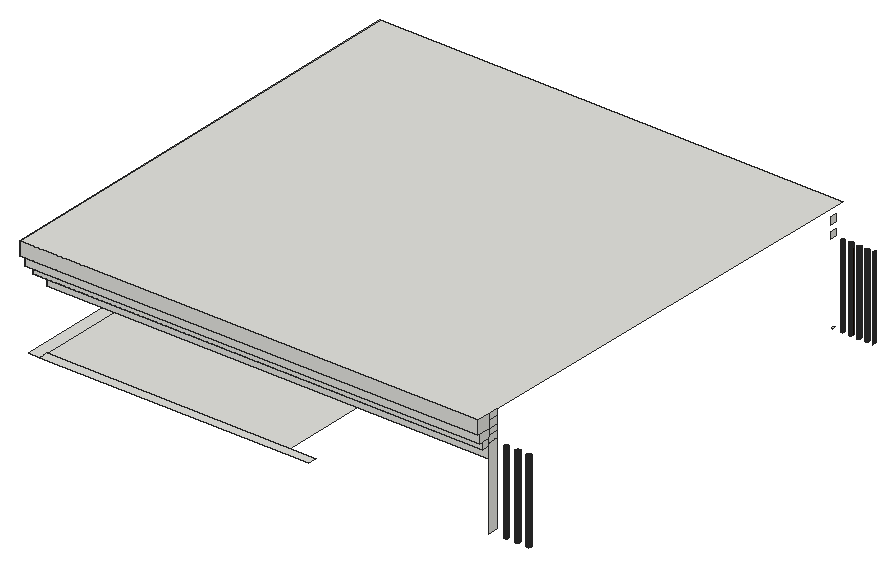
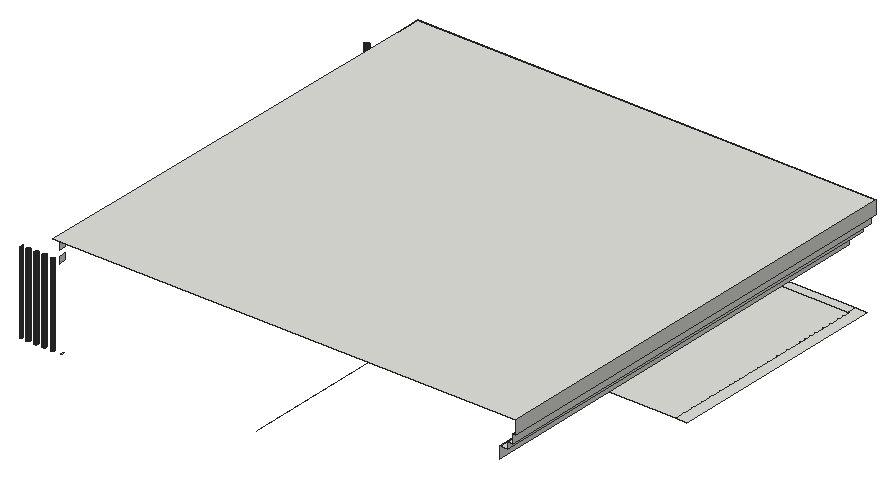
# SketchUp Ruby script. Lengths in inches.
U = 1.inch
M = Sketchup.active_model
def pt(a) = Geom::Point3d.new(a.map { |v| v * U })
def face(e, loops, mat)
  f = e.add_face(loops[0].map { |a| pt(a) })
  loops[1..].each { |l| e.add_face(l.map { |a| pt(a) }).erase! }
  f.material = f.back_material = mat if mat
  f
end
# faces: each face lists its corners as indices into pts; further lists are holes
def faces(e, pts, list, mat = nil) = list.each { |f| face(e, (f[0].is_a?(Array) ? f : [f]).map { |l| l.map { |i| pts[i] } }, mat) }
# xy, xz, yz: faces in a plane at the given z, y or x. An outline is a flat list of corners, or four numbers for a rectangle; further outlines are holes
def ring(l) = l.size == 4 ? [[l[0], l[1]], [l[2], l[1]], [l[2], l[3]], [l[0], l[3]]] : l.each_slice(2).to_a
def flat(e, list, mat, &to3) = list.each { |f| face(e, (f[0].is_a?(Array) ? f : [f]).map { |l| ring(l).map { |u, v| to3.(u, v) } }, mat) }
def xy(e, z, list, mat = nil) = flat(e, list, mat) { |x, y| [x, y, z] }
def xz(e, y, list, mat = nil) = flat(e, list, mat) { |x, z| [x, y, z] }
def yz(e, x, list, mat = nil) = flat(e, list, mat) { |y, z| [x, y, z] }
def lines(e, pts, list) = list.each { |a, b| e.add_line(pt(pts[a]), pt(pts[b])) }
# prism: a flat outline (further loops are holes) pulled along v
def prism(e, loops, v, mat = nil)
  f = face(e, loops, mat); d = Geom::Vector3d.new(v.map { |x| x * U })
  f.pushpull(f.normal.samedirection?(d) ? d.length : -d.length)
end
def box(e, o, s, mat = nil) = prism(e, [[o, [o[0] + s[0], o[1], o[2]], [o[0] + s[0], o[1] + s[1], o[2]], [o[0], o[1] + s[1], o[2]]]], [0, 0, s[2]], mat)
def at(x, y, z, deg = 0) = Geom::Transformation.translation(pt([x, y, z])) * Geom::Transformation.rotation(ORIGIN, Z_AXIS, deg.degrees)
def axes(o, x, y, z) = Geom::Transformation.new([*x, 0, *y, 0, *z, 0, *pt(o).to_a, 1])
def part(name) = M.definitions.add(name)
# library, detail: a bought-in or finely detailed component or shape, given as its bounding box
def library(name, o, s) = part(name).tap { |d| box(d.entities, o, s) }
def detail(e, o, s) = box(e.add_group.entities, o, s)
def put(e, d, t, mat = nil) = e.add_instance(d, t).tap { |i| i.material = mat if mat }
def group(e, t, mat = nil) = e.add_group.tap { |g| g.transformation = t; g.material = mat if mat }.entities
root = M.entities
M.materials.add("[Metal Seamed]1").color = [28, 14, 0]
xy(root,618.25,[[284.2,68.79,283.86,68.83,283.54,68.97,283.27,69.17,283.0625,69.45,282.93,69.76,282.89,70.1,282.93,70.44,283.0625,70.76,283.27,71.03,283.54,71.24,283.86,71.37,284.2,71.41,284.54,71.37,284.86,71.24,285.13,71.03,285.34,70.76,285.47,70.44,285.51,70.1,285.47,69.76,285.34,69.45,285.13,69.17,284.86,68.97,284.54,68.83],[290.89,68.79,290.55,68.83,290.23,68.97,289.96,69.17,289.75,69.45,289.62,69.76,289.57,70.1,289.62,70.44,289.75,70.76,289.96,71.03,290.23,71.24,290.55,71.37,290.89,71.41,291.23,71.37,291.54,71.24,291.81,71.03,292.02,70.76,292.15,70.44,292.2,70.1,292.15,69.76,292.02,69.45,291.81,69.17,291.54,68.97,291.23,68.83],[297.57,68.79,297.23,68.83,296.92,68.97,296.65,69.17,296.4375,69.45,296.31,69.76,296.26,70.1,296.31,70.44,296.4375,70.76,296.65,71.03,296.92,71.24,297.23,71.37,297.57,71.41,297.91,71.37,298.23,71.24,298.5,71.03,298.71,70.76,298.84,70.44,298.89,70.1,298.84,69.76,298.71,69.45,298.5,69.17,298.23,68.97,297.91,68.83],[284.08,318.74,283.8,318.8125,283.54,318.95,283.32,319.15,283.17,319.4,283.09,319.6875,283.08,319.98,283.15,320.27,283.29,320.52,283.49,320.74,283.74,320.89,284.02,320.97,284.32,320.98,284.6,320.91,284.86,320.77,285.07,320.57,285.23,320.32,285.31,320.04,285.32,319.74,285.25,319.46,285.11,319.2,284.91,318.99,284.66,318.83,284.375,318.75],[288.89,318.74,288.61,318.8125,288.35,318.95,288.14,319.15,287.98,319.4,287.9,319.6875,287.89,319.98,287.96,320.27,288.1,320.52,288.3,320.74,288.55,320.89,288.84,320.97,289.13,320.98,289.41,320.91,289.67,320.77,289.89,320.57,290.04,320.32,290.12,320.04,290.13,319.74,290.0625,319.46,289.92,319.2,289.72,318.99,289.47,318.83,289.1875,318.75],
  [293.71,318.74,293.42,318.8125,293.16,318.95,292.95,319.15,292.8,319.4,292.71,319.6875,292.71,319.98,292.77,320.27,292.91,320.52,293.12,320.74,293.37,320.89,293.65,320.97,293.94,320.98,294.23,320.91,294.49,320.77,294.7,320.57,294.85,320.32,294.94,320.04,294.94,319.74,294.875,319.46,294.73,319.2,294.53,318.99,294.28,318.83,294,318.75],[298.52,318.74,298.23,318.8125,297.98,318.95,297.76,319.15,297.61,319.4,297.53,319.6875,297.52,319.98,297.59,320.27,297.73,320.52,297.93,320.74,298.18,320.89,298.46,320.97,298.75,320.98,299.04,320.91,299.3,320.77,299.51,320.57,299.66,320.32,299.75,320.04,299.76,319.74,299.6875,319.46,299.55,319.2,299.34,318.99,299.09,318.83,298.8125,318.75],[278.79,318.92,278.8125,320.82,278.68,320.74,278.48,320.52,278.34,320.27,278.27,319.98,278.28,319.6875,278.36,319.4,278.51,319.15,278.73,318.95]])
xy(root,622.25,[[6.875,62.22,13.375,195.41],[13.375,62.22,173.1875,67.28],[13.375,67.28,158,195.41]])
xy(root,665,[[8.6875,62.97,13.375,326.53],[13.375,62.97,275.92,67.28]])
xy(root,666.9375,[[288.89,318.74,289.1875,318.75,289.47,318.83,289.72,318.99,289.92,319.2,290.0625,319.46,290.13,319.74,290.12,320.04,290.04,320.32,289.89,320.57,289.67,320.77,289.41,320.91,289.13,320.98,288.84,320.97,288.55,320.89,288.3,320.74,288.1,320.52,287.96,320.27,287.89,319.98,287.9,319.6875,287.98,319.4,288.14,319.15,288.35,318.95,288.61,318.8125]])
xy(root,669.0625,[[5.625,60.72,5.625,326.53,8.6875,326.53,8.6875,62.97,13.375,62.97,13.375,60.72],[13.375,60.72,275.92,62.97]])
xy(root,674.375,[[3.625,59.41,3.625,326.53,5.625,326.53,5.625,60.72,13.375,60.72,13.375,59.41],[13.375,59.41,275.92,60.72]])
xy(root,682.25,[[3.625,59.41,275.92,59.41,275.92,73.28,278.88,326.53,3.625,326.53]])
xz(root,59.41,[[3.625,674.375,275.92,682.25]])
xz(root,60.72,[[5.625,669.0625,275.92,674.375]])
xz(root,62.97,[[8.6875,665,275.92,669.0625]])
xz(root,67.28,[[13.375,658.25,275.92,665]])
yz(root,3.625,[[59.41,674.375,326.53,682.25]])
yz(root,5.625,[[60.72,669.0625,326.53,674.375]])
yz(root,8.6875,[[62.97,665,326.53,669.0625]])
yz(root,13.375,[[67.28,658.25,326.53,665]])
yz(root,275.92,[[67.28,618.25,73.28,666.66],[62.97,665,67.28,665,67.28,666.66,67.16,666.66,67.16,669.0625,62.97,669.0625],[67.16,666.66,73.28,670.37],[60.72,669.0625,67.16,669.0625,67.16,670.37,67.28,670.37,67.28,674.375,60.72,674.375],[67.28,670.37,73.28,674.375],
  [59.41,674.375,67.28,682.25],[67.28,674.375,73.28,678.3125],[67.28,678.3125,73.28,682.25]])
yz(root,278.82,[[317.52,674.05,321.28,678.3125]])
yz(root,278.88,[[317.52,666.66,321.28,670.37]])
yz(root,292.71,[[319.6875,618.25,319.98,666.66]],"[Metal Seamed]1")
yz(root,294.94,[[319.74,618.25,320.04,666.66]],"[Metal Seamed]1")
p = [[283.54,68.97,618.25],[283.86,68.83,618.25],[283.86,68.83,666.66],[283.54,68.97,666.66],[284.2,68.79,618.25],[284.2,68.79,666.66],
  [284.54,68.83,618.25],[284.54,68.83,666.66],[284.86,68.97,618.25],[284.86,68.97,666.66],[290.23,68.97,618.25],[290.55,68.83,618.25],
  [290.55,68.83,666.66],[290.23,68.97,666.66],[290.89,68.79,618.25],[290.89,68.79,666.66],[291.23,68.83,618.25],[291.23,68.83,666.66],
  [291.54,68.97,618.25],[291.54,68.97,666.66],[296.92,68.97,618.25],[297.23,68.83,618.25],[297.23,68.83,666.66],[296.92,68.97,666.66],
  [297.57,68.79,618.25],[297.57,68.79,666.66],[297.91,68.83,618.25],[297.91,68.83,666.66],[298.23,68.97,618.25],[298.23,68.97,666.66],
  [283.27,69.17,618.25],[283.27,69.17,666.66],[285.13,69.17,618.25],[285.13,69.17,666.66],[289.96,69.17,618.25],[289.96,69.17,666.66],
  [291.81,69.17,618.25],[291.81,69.17,666.66],[296.65,69.17,618.25],[296.65,69.17,666.66],[298.5,69.17,618.25],[298.5,69.17,666.66],
  [283.0625,69.45,618.25],[283.0625,69.45,666.66],[285.34,69.45,618.25],[285.34,69.45,666.66],[289.75,69.45,618.25],[289.75,69.45,666.66],
  [292.02,69.45,618.25],[292.02,69.45,666.66],[296.4375,69.45,618.25],[296.4375,69.45,666.66],[298.71,69.45,618.25],[298.71,69.45,666.66],
  [282.93,69.76,618.25],[282.93,69.76,666.66],[285.47,69.76,618.25],[285.47,69.76,666.66],[289.62,69.76,618.25],[289.62,69.76,666.66],
  [292.15,69.76,618.25],[292.15,69.76,666.66],[296.31,69.76,618.25],[296.31,69.76,666.66],[298.84,69.76,618.25],[298.84,69.76,666.66],
  [282.89,70.1,618.25],[282.89,70.1,666.66],[285.51,70.1,618.25],[285.51,70.1,666.66],[289.57,70.1,618.25],[289.57,70.1,666.66],
  [292.2,70.1,618.25],[292.2,70.1,666.66],[296.26,70.1,618.25],[296.26,70.1,666.66],[298.89,70.1,618.25],[298.89,70.1,666.66],
  [282.93,70.44,618.25],[282.93,70.44,666.66],[285.47,70.44,618.25],[285.47,70.44,666.66],[289.62,70.44,618.25],[289.62,70.44,666.66],
  [292.15,70.44,618.25],[292.15,70.44,666.66],[296.31,70.44,618.25],[296.31,70.44,666.66],[298.84,70.44,618.25],[298.84,70.44,666.66],
  [283.0625,70.76,618.25],[283.0625,70.76,666.66],[285.34,70.76,618.25],[285.34,70.76,666.66],[289.75,70.76,618.25],[289.75,70.76,666.66],
  [292.02,70.76,618.25],[292.02,70.76,666.66],[296.4375,70.76,618.25],[296.4375,70.76,666.66],[298.71,70.76,618.25],[298.71,70.76,666.66],
  [283.27,71.03,618.25],[283.27,71.03,666.66],[285.13,71.03,618.25],[285.13,71.03,666.66],[289.96,71.03,618.25],[289.96,71.03,666.66],
  [291.81,71.03,618.25],[291.81,71.03,666.66],[296.65,71.03,618.25],[296.65,71.03,666.66],[298.5,71.03,618.25],[298.5,71.03,666.66],
  [283.54,71.24,618.25],[283.54,71.24,666.66],[284.86,71.24,618.25],[284.86,71.24,666.66],[290.23,71.24,618.25],[290.23,71.24,666.66],
  [291.54,71.24,618.25],[291.54,71.24,666.66],[296.92,71.24,618.25],[296.92,71.24,666.66],[298.23,71.24,618.25],[298.23,71.24,666.66],
  [283.86,71.37,618.25],[283.86,71.37,666.66],[284.54,71.37,618.25],[284.54,71.37,666.66],[290.55,71.37,618.25],[290.55,71.37,666.66],
  [291.23,71.37,618.25],[291.23,71.37,666.66],[297.23,71.37,618.25],[297.23,71.37,666.66],[297.91,71.37,618.25],[297.91,71.37,666.66],
  [284.2,71.41,618.25],[284.2,71.41,666.66],[290.89,71.41,618.25],[290.89,71.41,666.66],[297.57,71.41,618.25],[297.57,71.41,666.66],
  [283.8,318.8125,618.25],[284.08,318.74,618.25],[284.08,318.74,666.66],[283.8,318.8125,666.66],[284.375,318.75,618.25],[284.375,318.75,666.66],
  [288.61,318.8125,618.25],[288.89,318.74,618.25],[288.89,318.74,666.9375],[288.61,318.8125,666.9375],[289.1875,318.75,618.25],[289.1875,318.75,666.9375],
  [293.42,318.8125,618.25],[293.71,318.74,618.25],[293.71,318.74,666.66],[293.42,318.8125,666.66],[294,318.75,618.25],[294,318.75,666.66],
  [298.23,318.8125,618.25],[298.52,318.74,618.25],[298.52,318.74,666.66],[298.23,318.8125,666.66],[298.8125,318.75,618.25],[298.8125,318.75,666.66],
  [283.54,318.95,618.25],[283.54,318.95,666.66],[284.66,318.83,618.25],[284.66,318.83,666.66],[284.91,318.99,618.25],[284.91,318.99,666.66],
  [288.35,318.95,618.25],[288.35,318.95,666.9375],[289.47,318.83,618.25],[289.47,318.83,666.9375],[289.72,318.99,618.25],[289.72,318.99,666.9375],
  [293.16,318.95,618.25],[293.16,318.95,666.66],[294.28,318.83,618.25],[294.28,318.83,666.66],[294.53,318.99,618.25],[294.53,318.99,666.66],
  [297.98,318.95,618.25],[297.98,318.95,666.66],[299.09,318.83,618.25],[299.09,318.83,666.66],[299.34,318.99,618.25],[299.34,318.99,666.66],
  [302.79,318.95,618.25],[303.05,318.8125,618.25],[303.05,318.8125,666.9375],[302.79,318.95,666.9375],[283.32,319.15,618.25],[283.32,319.15,666.66],
  [285.11,319.2,618.25],[285.11,319.2,666.66],[288.14,319.15,618.25],[288.14,319.15,666.9375],[289.92,319.2,618.25],[289.92,319.2,666.9375],
  [292.95,319.15,618.25],[292.95,319.15,666.66],[294.73,319.2,618.25],[294.73,319.2,666.66],[297.76,319.15,618.25],[297.76,319.15,666.66],
  [299.55,319.2,618.25],[299.55,319.2,666.66],[302.57,319.15,618.25],[302.57,319.15,666.9375],[283.17,319.4,618.25],[283.17,319.4,666.66],
  [285.25,319.46,618.25],[285.25,319.46,666.66],[287.98,319.4,618.25],[287.98,319.4,666.9375],[290.0625,319.46,618.25],[290.0625,319.46,666.9375],
  [292.8,319.4,618.25],[292.8,319.4,666.66],[294.875,319.46,618.25],[294.875,319.46,666.66],[297.61,319.4,618.25],[297.61,319.4,666.66],
  [299.6875,319.46,618.25],[299.6875,319.46,666.66],[302.42,319.4,618.25],[302.42,319.4,666.9375],[283.09,319.6875,618.25],[283.09,319.6875,666.66],
  [287.9,319.6875,618.25],[287.9,319.6875,666.9375],[292.71,319.6875,618.25],[292.71,319.6875,666.66],[297.53,319.6875,618.25],[297.53,319.6875,666.66],
  [302.34,319.6875,618.25],[302.34,319.6875,666.9375],[285.32,319.74,618.25],[285.32,319.74,666.66],[290.13,319.74,618.25],[290.13,319.74,666.9375],
  [294.94,319.74,618.25],[294.94,319.74,666.66],[299.76,319.74,618.25],[299.76,319.74,666.66],[283.08,319.98,618.25],[283.08,319.98,666.66],
  [285.31,320.04,618.25],[285.31,320.04,666.66],[287.89,319.98,618.25],[287.89,319.98,666.9375],[290.12,320.04,618.25],[290.12,320.04,666.9375],
  [297.52,319.98,618.25],[297.52,319.98,666.66],[299.75,320.04,618.25],[299.75,320.04,666.66],[302.33,319.98,618.25],[302.33,319.98,666.9375],
  [283.15,320.27,618.25],[283.15,320.27,666.66],[285.23,320.32,618.25],[285.23,320.32,666.66],[287.96,320.27,618.25],[287.96,320.27,666.9375],
  [290.04,320.32,618.25],[290.04,320.32,666.9375],[292.77,320.27,618.25],[292.71,319.98,618.25],[292.71,319.98,666.66],[292.77,320.27,666.66],
  [294.94,320.04,618.25],[294.85,320.32,618.25],[294.85,320.32,666.66],[294.94,320.04,666.66],[297.59,320.27,618.25],[297.59,320.27,666.66],
  [299.66,320.32,618.25],[299.66,320.32,666.66],[302.4,320.27,618.25],[302.4,320.27,666.9375],[283.29,320.52,618.25],[283.29,320.52,666.66],
  [285.07,320.57,618.25],[285.07,320.57,666.66],[288.1,320.52,618.25],[288.1,320.52,666.9375],[289.89,320.57,618.25],[289.89,320.57,666.9375],
  [292.91,320.52,618.25],[292.91,320.52,666.66],[294.7,320.57,618.25],[294.7,320.57,666.66],[297.73,320.52,618.25],[297.73,320.52,666.66],
  [299.51,320.57,618.25],[299.51,320.57,666.66],[302.54,320.52,618.25],[302.54,320.52,666.9375],[283.49,320.74,618.25],[283.49,320.74,666.66],
  [288.3,320.74,618.25],[288.3,320.74,666.9375],[293.12,320.74,618.25],[293.12,320.74,666.66],[297.93,320.74,618.25],[297.93,320.74,666.66],
  [302.74,320.74,618.25],[302.74,320.74,666.9375],[284.86,320.77,618.25],[284.86,320.77,666.66],[289.67,320.77,618.25],[289.67,320.77,666.9375],
  [294.49,320.77,618.25],[294.49,320.77,666.66],[299.3,320.77,618.25],[299.3,320.77,666.66],[283.74,320.89,618.25],[283.74,320.89,666.66],
  [288.55,320.89,618.25],[288.55,320.89,666.9375],[293.37,320.89,618.25],[293.37,320.89,666.66],[298.18,320.89,618.25],[298.18,320.89,666.66],
  [302.99,320.89,618.25],[302.99,320.89,666.9375],[284.6,320.91,618.25],[284.6,320.91,666.66],[289.41,320.91,618.25],[289.41,320.91,666.9375],
  [294.23,320.91,618.25],[294.23,320.91,666.66],[299.04,320.91,618.25],[299.04,320.91,666.66],[284.02,320.97,618.25],[284.02,320.97,666.66],
  [284.32,320.98,618.25],[284.32,320.98,666.66],[288.84,320.97,618.25],[288.84,320.97,666.9375],[289.13,320.98,618.25],[289.13,320.98,666.9375],
  [293.65,320.97,618.25],[293.65,320.97,666.66],[293.94,320.98,618.25],[293.94,320.98,666.66],[298.46,320.97,618.25],[298.46,320.97,666.66],
  [298.75,320.98,618.25],[298.75,320.98,666.66],[158,195.41,622.25],[158,326.53,622.25],[158,195.41,658.25]]
faces(root,p,[[0,1,2,3],[1,4,5,2],[4,6,7,5],[6,8,9,7],[10,11,12,13],[11,14,15,12],[14,16,17,15],[16,18,19,17],
  [20,21,22,23],[21,24,25,22],[24,26,27,25],[26,28,29,27],[30,0,3,31],[8,32,33,9],[34,10,13,35],[18,36,37,19],
  [38,20,23,39],[28,40,41,29],[42,30,31,43],[32,44,45,33],[46,34,35,47],[36,48,49,37],[50,38,39,51],[40,52,53,41],
  [54,42,43,55],[44,56,57,45],[58,46,47,59],[48,60,61,49],[62,50,51,63],[52,64,65,53],[66,54,55,67],[56,68,69,57],
  [70,58,59,71],[60,72,73,61],[74,62,63,75],[64,76,77,65],[78,66,67,79],[68,80,81,69],[82,70,71,83],[72,84,85,73],
  [86,74,75,87],[76,88,89,77],[90,78,79,91],[80,92,93,81],[94,82,83,95],[84,96,97,85],[98,86,87,99],[88,100,101,89],
  [102,90,91,103],[92,104,105,93],[106,94,95,107],[96,108,109,97],[110,98,99,111],[100,112,113,101],[114,102,103,115],[104,116,117,105],
  [118,106,107,119],[108,120,121,109],[122,110,111,123],[112,124,125,113],[126,114,115,127],[116,128,129,117],[130,118,119,131],[120,132,133,121],
  [134,122,123,135],[124,136,137,125],[138,126,127,139],[128,138,139,129],[140,130,131,141],[132,140,141,133],[142,134,135,143],[136,142,143,137],
  [144,145,146,147],[145,148,149,146],[150,151,152,153],[151,154,155,152],[156,157,158,159],[157,160,161,158],[162,163,164,165],[163,166,167,164],
  [168,144,147,169],[148,170,171,149],[170,172,173,171],[174,150,153,175],[154,176,177,155],[176,178,179,177],[180,156,159,181],[160,182,183,161],
  [182,184,185,183],[186,162,165,187],[166,188,189,167],[188,190,191,189],[192,193,194,195],[196,168,169,197],[172,198,199,173],[200,174,175,201],
  [178,202,203,179],[204,180,181,205],[184,206,207,185],[208,186,187,209],[190,210,211,191],[212,192,195,213],[214,196,197,215],[198,216,217,199],
  [218,200,201,219],[202,220,221,203],[222,204,205,223],[206,224,225,207],[226,208,209,227],[210,228,229,211],[230,212,213,231],[232,214,215,233],
  [234,218,219,235],[236,222,223,237],[238,226,227,239],[240,230,231,241],[216,242,243,217],[220,244,245,221],[224,246,247,225],[228,248,249,229],
  [250,232,233,251],[242,252,253,243],[254,234,235,255],[244,256,257,245],[258,238,239,259],[248,260,261,249],[262,240,241,263],[264,250,251,265],
  [252,266,267,253],[268,254,255,269],[256,270,271,257],[272,273,274,275],[276,277,278,279],[280,258,259,281],[260,282,283,261],[284,262,263,285],
  [286,264,265,287],[266,288,289,267],[290,268,269,291],[270,292,293,271],[294,272,275,295],[277,296,297,278],[298,280,281,299],[282,300,301,283],
  [302,284,285,303],[304,286,287,305],[306,290,291,307],[308,294,295,309],[310,298,299,311],[312,302,303,313],[288,314,315,289],[292,316,317,293],
  [296,318,319,297],[300,320,321,301],[322,304,305,323],[324,306,307,325],[326,308,309,327],[328,310,311,329],[330,312,313,331],[314,332,333,315],
  [316,334,335,317],[318,336,337,319],[320,338,339,321],[340,322,323,341],[332,342,343,333],[344,324,325,345],[334,346,347,335],[348,326,327,349],
  [336,350,351,337],[352,328,329,353],[338,354,355,339],[342,340,341,343],[346,344,345,347],[350,348,349,351],[354,352,353,355]],"[Metal Seamed]1")
lines(root,p,[[356,357],[356,358]])
